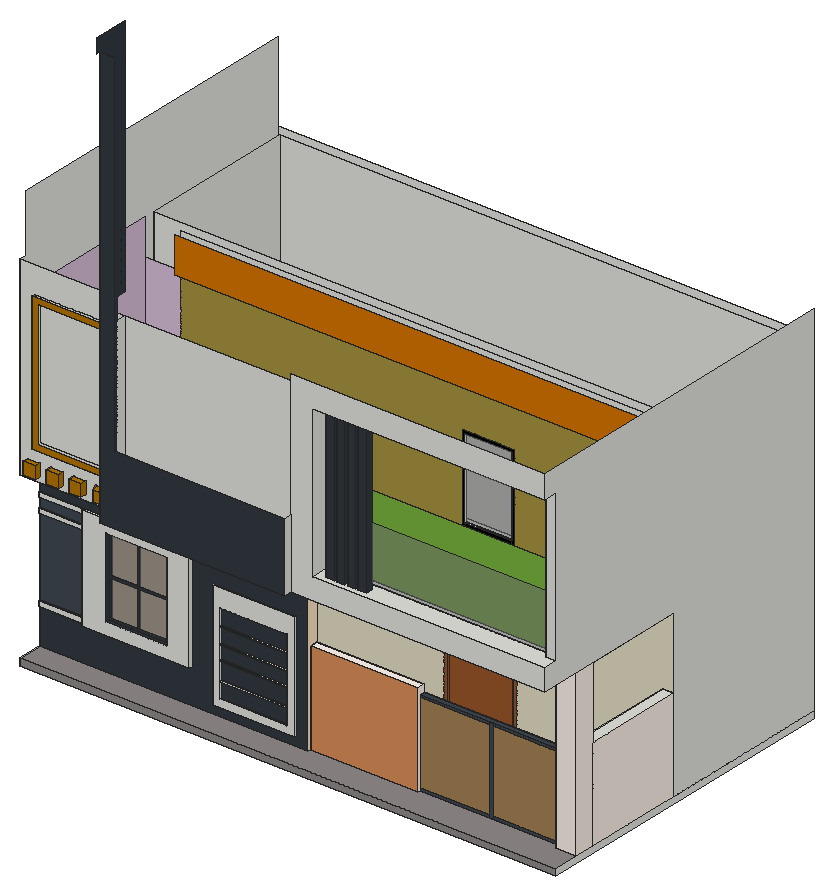
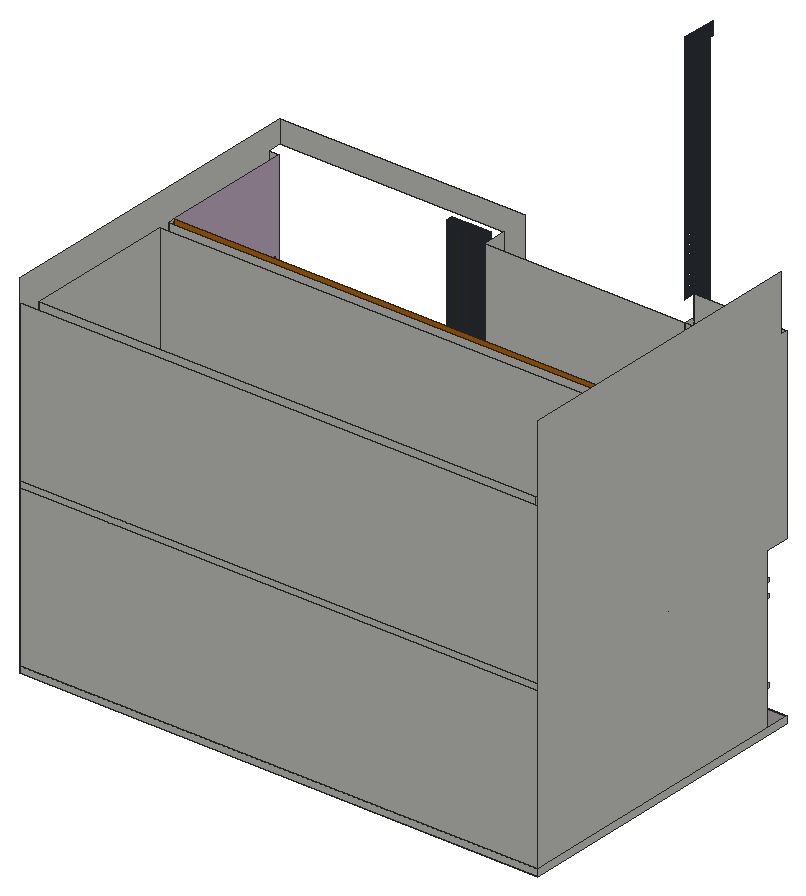
# SketchUp Ruby script. Lengths in inches.
U = 1.inch
M = Sketchup.active_model
def pt(a) = Geom::Point3d.new(a.map { |v| v * U })
def face(e, loops, mat)
  f = e.add_face(loops[0].map { |a| pt(a) })
  loops[1..].each { |l| e.add_face(l.map { |a| pt(a) }).erase! }
  f.material = f.back_material = mat if mat
  f
end
# faces: each face lists its corners as indices into pts; further lists are holes
def faces(e, pts, list, mat = nil) = list.each { |f| face(e, (f[0].is_a?(Array) ? f : [f]).map { |l| l.map { |i| pts[i] } }, mat) }
# xy, xz, yz: faces in a plane at the given z, y or x. An outline is a flat list of corners, or four numbers for a rectangle; further outlines are holes
def ring(l) = l.size == 4 ? [[l[0], l[1]], [l[2], l[1]], [l[2], l[3]], [l[0], l[3]]] : l.each_slice(2).to_a
def flat(e, list, mat, &to3) = list.each { |f| face(e, (f[0].is_a?(Array) ? f : [f]).map { |l| ring(l).map { |u, v| to3.(u, v) } }, mat) }
def xy(e, z, list, mat = nil) = flat(e, list, mat) { |x, y| [x, y, z] }
def xz(e, y, list, mat = nil) = flat(e, list, mat) { |x, z| [x, y, z] }
def yz(e, x, list, mat = nil) = flat(e, list, mat) { |y, z| [x, y, z] }
def lines(e, pts, list) = list.each { |a, b| e.add_line(pt(pts[a]), pt(pts[b])) }
# prism: a flat outline (further loops are holes) pulled along v
def prism(e, loops, v, mat = nil)
  f = face(e, loops, mat); d = Geom::Vector3d.new(v.map { |x| x * U })
  f.pushpull(f.normal.samedirection?(d) ? d.length : -d.length)
end
def box(e, o, s, mat = nil) = prism(e, [[o, [o[0] + s[0], o[1], o[2]], [o[0] + s[0], o[1] + s[1], o[2]], [o[0], o[1] + s[1], o[2]]]], [0, 0, s[2]], mat)
def at(x, y, z, deg = 0) = Geom::Transformation.translation(pt([x, y, z])) * Geom::Transformation.rotation(ORIGIN, Z_AXIS, deg.degrees)
def axes(o, x, y, z) = Geom::Transformation.new([*x, 0, *y, 0, *z, 0, *pt(o).to_a, 1])
def part(name) = M.definitions.add(name)
# library, detail: a bought-in or finely detailed component or shape, given as its bounding box
def library(name, o, s) = part(name).tap { |d| box(d.entities, o, s) }
def detail(e, o, s) = box(e.add_group.entities, o, s)
def put(e, d, t, mat = nil) = e.add_instance(d, t).tap { |i| i.material = mat if mat }
def group(e, t, mat = nil) = e.add_group.tap { |g| g.transformation = t; g.material = mat if mat }.entities
root = M.entities
M.materials.add("[0009_Linen]").color = [250, 240, 230]
M.materials.add("[0011_Seashell]").color = [255, 245, 238]
M.materials.add("[0012_Bisque]").color = [186, 166, 143]
M.materials.add("[0012_Bisque]1").color = [255, 228, 196]
M.materials.add("[0038_Orange]").color = [181, 117, 0]
M.materials.add("[0039_DarkOrange]").color = [214, 117, 0]
M.materials.add("[0051_Cornsilk]").color = [226, 220, 195]
M.materials.add("[0111_SlateGray]").color = [51, 58, 66]
M.materials.add("[0111_SlateGray]2").color = [63, 72, 81]
M.materials.add("[0116_Lavender]").color = [230, 230, 250]
M.materials.add("[0118_Thistle]").color = [216, 191, 216]
M.materials.add("[0137_Black]").color = [0, 0, 0]
M.materials.add("[Beadboard]").color = [218, 143, 90]
M.materials.add("[Granite Brown]").color = [126, 104, 91]
M.materials.add("[Grass Dark Green]").color = [106, 157, 55]
M.materials.add("[Modern Siding]").color = [163, 129, 83]
M.materials.add("[Stone Coursed Rough]").color = [165, 147, 63]
M.materials.add("[Stone Marble]").color = [143, 138, 136]
M.materials.add("[Translucent Glass Gray]").color = [128, 128, 128]
M.materials["[Translucent Glass Gray]"].alpha = 0.5
M.materials.add("[Wood Cherry Original]").color = [152, 86, 42]
xy(root,0,[[0,138,900,678]])
xy(root,12,[[0,180,18,396],[18,180,450,198],[865.875,180,900,214.125],[450,185,630,198],[630,189,865.875,198],
  [882,214.125,900,384],[882,384,882,660,18,660,18,396,0,396,0,678,900,678,900,384],[18,384,882,396],[18,396,882,660]])
xy(root,12,[[18,198,865.875,198,865.875,214.125,882,214.125,882,384,18,384]],"[Granite Brown]")
xy(root,12,[[0,138,900,138,900,180,865.875,180,865.875,189,630,189,630,185,450,185,450,180,0,180]],"[Stone Marble]")
xy(root,19.46,[[521.75,384,630.34,386]],"[Wood Cherry Original]")
xy(root,27.77,[[292.08,177,429.33,180]])
xy(root,39.77,[[304.08,177,417.33,180]])
xy(root,66.37,[[304.08,177,417.33,180]])
xy(root,68.32,[[304.08,177,417.33,180]])
xy(root,70.46,[[74.4,174,254.15,180]])
xy(root,73.28,[[0,177,74.4,180]])
xy(root,81.37,[[0,177,74.4,180]])
xy(root,91.52,[[115.89,174,217.33,180]],"[0111_SlateGray]")
xy(root,96.88,[[304.08,177,417.33,180]])
xy(root,98.83,[[304.08,177,417.33,180]])
xy(root,121.13,[[304.08,177,417.33,180]])
xy(root,123.08,[[304.08,177,417.33,180]])
xy(root,148.13,[[304.08,177,417.33,180]])
xy(root,150.08,[[304.08,177,417.33,180]])
xy(root,156,[[630,189,865.875,198]],"[0111_SlateGray]2")
xy(root,168,[[882,214.125,900,384]])
xy(root,168,[[450,185,630,198]],"[0011_Seashell]")
xy(root,177.77,[[304.08,177,417.33,180]])
xy(root,204.37,[[521.75,384,630.34,386]],"[Wood Cherry Original]")
xy(root,207.77,[[292.08,177,429.33,180]])
xy(root,213.2,[[0,177,74.4,180]])
xy(root,220.36,[[0,177,74.4,180]])
xy(root,224.58,[[115.89,174,217.33,180]],"[0111_SlateGray]")
xy(root,237.75,[[0,177,74.4,180]])
xy(root,244.84,[[74.4,174,254.15,180],[0,177,74.4,180]])
xy(root,288,[[18,384,882,396],[18,396,882,660]])
xy(root,288,[[[162,102,162,138,0,138,0,180,450,180,450,198,18,198,18,384,900,384,900,214.125,865.875,214.125,865.875,180,900,180,900,114,474,114,474,102],[627.41,194.94,630.54,194.97,633.5625,195.81,636.26,197.39,638.46,199.63,640,202.35,640.79,205.39,640.76,208.52,639.93,211.54,638.34,214.24,636.1,216.43,633.38,217.98,630.35,218.76,627.21,218.74,624.19,217.9,621.49,216.3125,619.3,214.08,617.75,211.36,616.97,208.32,616.99,205.19,617.83,202.17,619.42,199.47,621.65,197.27,624.375,195.73],[507.41,194.94,510.54,194.97,513.5625,195.81,516.26,197.39,518.46,199.63,520,202.35,520.79,205.39,520.76,208.52,519.93,211.54,518.34,214.24,516.1,216.43,513.38,217.98,510.35,218.76,507.21,218.74,504.19,217.9,501.49,216.3125,499.3,214.08,497.75,211.36,496.97,208.32,496.99,205.19,497.83,202.17,499.42,199.47,501.65,197.27,504.375,195.73],[747.41,194.94,750.54,194.97,753.5625,195.81,756.26,197.39,758.46,199.63,760,202.35,760.79,205.39,760.76,208.52,759.93,211.54,758.34,214.24,756.1,216.43,753.38,217.98,750.35,218.76,747.21,218.74,744.19,217.9,741.49,216.3125,739.3,214.08,737.75,211.36,736.97,208.32,736.99,205.19,737.83,202.17,739.42,199.47,741.65,197.27,744.375,195.73]],[507.41,194.94,504.375,195.73,501.65,197.27,499.42,199.47,497.83,202.17,496.99,205.19,496.97,208.32,497.75,211.36,499.3,214.08,501.49,216.3125,504.19,217.9,507.21,218.74,510.35,218.76,513.38,217.98,516.1,216.43,518.34,214.24,519.93,211.54,520.76,208.52,520.79,205.39,520,202.35,518.46,199.63,516.26,197.39,513.5625,195.81,510.54,194.97],[627.41,194.94,624.375,195.73,621.65,197.27,619.42,199.47,617.83,202.17,616.99,205.19,616.97,208.32,617.75,211.36,619.3,214.08,621.49,216.3125,624.19,217.9,627.21,218.74,630.35,218.76,633.38,217.98,636.1,216.43,638.34,214.24,639.93,211.54,640.76,208.52,640.79,205.39,640,202.35,638.46,199.63,636.26,197.39,633.5625,195.81,630.54,194.97],[747.41,194.94,744.375,195.73,741.65,197.27,739.42,199.47,737.83,202.17,736.99,205.19,736.97,208.32,737.75,211.36,739.3,214.08,741.49,216.3125,744.19,217.9,747.21,218.74,750.35,218.76,753.38,217.98,756.1,216.43,758.34,214.24,759.93,211.54,760.76,208.52,760.79,205.39,760,202.35,758.46,199.63,756.26,197.39,753.5625,195.81,750.54,194.97]],"[0116_Lavender]")
xy(root,296.37,[[12.68,129,33.18,138],[51.08,129,71.58,138],[89.48,129,109.98,138],[129.52,129,127.875,138,148.375,138,148.375,129]],"[0038_Orange]")
xy(root,300,[[822,366,882,378],[18,396,882,660]])
xy(root,300,[[18,156,882,156,882,366,822,366,822,378,18,378]],"[Grass Dark Green]")
xy(root,305.36,[[554.68,378,633.07,380]])
xy(root,316.87,[[12.68,129,33.18,138],[51.08,129,71.58,138],[89.48,129,109.98,138]],"[0038_Orange]")
xy(root,324,[[[510,114,900,114,900,138,882,138,882,147,510,147],[524.46,124.29,538.65,136.29],[542.46,124.29,556.65,136.29],[560.46,124.29,574.65,136.29],[578.46,124.29,592.65,136.29]],[524.46,124.29,538.65,136.29],[542.46,124.29,556.65,136.29],[560.46,124.29,574.65,136.29],[578.46,124.29,592.65,136.29],
  [510,147,882,156]])
xy(root,338.14,[[25.18,132,152.37,138]],"[0038_Orange]")
xz(root,102,[[162,288,474,288,474,404.14,186,404.14,186,996,162,996]],"[0111_SlateGray]")
xz(root,114,[[474,288,900,288,900,324,510,324,510,576,900,576,900,615.875,474,615.875]])
xz(root,124.29,[[524.46,324,538.65,576],[542.46,324,556.65,576],[560.46,324,574.65,576],[578.46,324,592.65,576]],"[0111_SlateGray]")
xz(root,129,[[12.68,296.37,33.18,316.87],[51.08,296.37,71.58,316.87],[89.48,296.37,109.98,316.87],[129.52,296.37,148.375,315.23]],"[0038_Orange]")
xz(root,132,[[[25.18,338.14,152.37,567.51],[34.01,346.96,143.55,558.6875]]],"[0038_Orange]")
xz(root,136.29,[[524.46,324,538.65,576],[542.46,324,556.65,576],[560.46,324,574.65,576],[578.46,324,592.65,576]],"[0111_SlateGray]")
xz(root,138,[[[0,288,162,612],[25.18,338.14,152.37,567.51],[12.68,296.37,33.18,316.87],[51.08,296.37,71.58,316.87],[89.48,296.37,109.98,316.87],[127.875,296.37,148.375,316.87]],[127.875,296.37,148.375,316.87],[882,324,900,576],[[25.18,338.14,152.37,567.51],[34.01,346.96,143.55,558.6875]]])
xz(root,138,[[0,0,900,12]],"[Stone Marble]")
xz(root,147,[[510,324,882,417]],"[Translucent Glass Gray]")
xz(root,156,[[18,300,162,576],[162,300,510,576],[510,300,882,324]])
xz(root,174,[[[74.4,70.46,254.15,244.84],[115.89,91.52,217.33,224.58]]])
xz(root,177,[[[292.08,27.77,429.33,207.77],[304.08,39.77,417.33,177.77]],[304.08,66.37,417.33,68.32],[0,73.28,74.4,81.37],[304.08,96.88,417.33,98.83],[304.08,121.13,417.33,123.08],
  [304.08,148.13,417.33,150.08],[0,213.2,74.4,220.36],[0,237.75,74.4,244.84]])
xz(root,180,[[[292.08,27.77,429.33,207.77],[304.08,39.77,417.33,177.77]],[[74.4,70.46,254.15,244.84],[115.89,91.52,217.33,224.58]],[0,73.28,74.4,81.37],[0,213.2,74.4,220.36],[0,237.75,74.4,244.84]])
xz(root,180,[[865.875,12,900,288]],"[0009_Linen]")
xz(root,180,[[[0,12,450,12,450,288,0,288,0,244.84,254.15,244.84,254.15,70.46,74.4,70.46,74.4,73.28,0,73.28],[292.08,27.77,429.33,207.77]],[304.08,39.77,417.33,66.37],[304.08,68.32,417.33,96.88],[[115.89,91.52,217.33,224.58],[119.83,95.46,213.38,220.64]],[164.78,95.46,168.08,155.49],
  [304.08,98.83,417.33,121.13],[304.08,123.08,417.33,148.13],[304.08,150.08,417.33,177.77],[119.83,155.49,164.78,159.39],[164.78,155.49,168.08,159.39],
  [168.08,155.49,213.38,159.39],[164.78,159.39,168.08,220.64]],"[0111_SlateGray]")
xz(root,180,[[0,81.37,74.4,213.2],[0,220.36,74.4,237.75]],"[0111_SlateGray]2")
xz(root,180,[[119.83,95.46,164.78,155.49],[168.08,95.46,213.38,155.49],[119.83,159.39,164.78,220.64],[168.08,159.39,213.38,220.64]],"[Translucent Glass Gray]")
xz(root,185,[[450,12,630,168]],"[Beadboard]")
xz(root,189,[[630,12,746.93,16.45],[746.93,12,752.1,156],[752.1,12,865.875,16.45],[630,151.97,746.93,156],[752.1,151.97,865.875,156]],"[0111_SlateGray]2")
xz(root,189,[[630,16.45,746.93,151.97],[752.1,16.45,865.875,151.97]],"[Modern Siding]")
xz(root,198,[[18,12,450,288]],"[0012_Bisque]")
xz(root,198,[[450,12,630,168]],"[Beadboard]")
xz(root,198,[[630,12,865.875,156]],"[Modern Siding]")
xz(root,214.125,[[882,12,900,168]])
xz(root,214.125,[[865.875,12,865.875,288,900,288,900,168,882,168,882,12]],"[0011_Seashell]")
xz(root,366,[[822,300,882,300,882,576,78,576,78,516,822,516]],"[0039_DarkOrange]")
xz(root,378,[[822,300,822,516,78,516,78,576,882,576,882,300]])
xz(root,378,[[18,300,78,516]],"[0118_Thistle]")
xz(root,378,[[549.3125,300,554.68,300,554.68,438.84,633.07,438.84,633.07,300,638.4375,300,638.4375,444.21,549.3125,444.21],[554.68,300,633.07,305.36]],"[0137_Black]")
xz(root,378,[[78,300,549.3125,300,549.3125,444.21,638.4375,444.21,638.4375,300,822,300,822,516,78,516]],"[Stone Coursed Rough]")
xz(root,380,[[554.68,305.36,633.07,438.84]],"[Translucent Glass Gray]")
xz(root,384,[[882,12,900,168]])
xz(root,384,[[18,12,514.29,12,514.29,211.83,637.79,211.83,637.79,12,882,12,882,168,900,168,900,288,18,288]],"[0051_Cornsilk]")
xz(root,384,[[[514.29,12,637.79,211.83],[521.75,19.46,630.34,204.37]]],"[Wood Cherry Original]")
xz(root,386,[[521.75,19.46,630.34,204.37]],"[Wood Cherry Original]")
xz(root,396,[[18,12,882,288],[18,300,882,576]])
xz(root,660,[[18,12,882,288],[18,300,882,576]])
xz(root,678,[[0,0,900,12],[0,12,900,288],[0,288,900,300],[0,300,900,576]])
yz(root,0,[[138,0,678,12],[180,12,180,288,138,288,138,612,149.68,612,149.68,709.65,678,709.65,678,12],[177,73.28,180,81.37],[177,213.2,180,220.36],[177,237.75,180,244.84]])
yz(root,12.68,[[129,296.37,138,316.87]],"[0038_Orange]")
yz(root,18,[[384,12,396,288],[396,12,660,288],[396,300,660,576]])
yz(root,18,[[198,12,384,288]],"[0012_Bisque]")
yz(root,18,[[156,300,378,576]],"[0118_Thistle]")
yz(root,25.18,[[132,338.14,138,567.51]],"[0038_Orange]")
yz(root,33.18,[[129,296.37,138,316.87]],"[0038_Orange]")
yz(root,51.08,[[129,296.37,138,316.87]],"[0038_Orange]")
yz(root,71.58,[[129,296.37,138,316.87]],"[0038_Orange]")
yz(root,74.4,[[174,70.46,174,244.84,177,244.84,177,237.75,180,237.75,180,220.36,177,220.36,177,213.2,180,213.2,180,81.37,177,81.37,177,73.28,180,73.28,180,70.46],[177,73.28,180,81.37],[177,213.2,180,220.36],[177,237.75,180,244.84]])
yz(root,89.48,[[129,296.37,138,316.87]],"[0038_Orange]")
yz(root,109.98,[[129,296.37,138,316.87]],"[0038_Orange]")
yz(root,115.89,[[174,91.52,180,224.58]],"[0111_SlateGray]")
yz(root,148.375,[[129,296.37,138,296.37,138,316.87,129,315.23]],"[0038_Orange]")
yz(root,152.37,[[132,338.14,138,567.51]],"[0038_Orange]")
yz(root,162,[[138,300,156,576]])
yz(root,162,[[[102,288,102,996,96,996,96,1020,156,1020,156,612,138,612,138,288],[146.77,660.69,147,660.7,147.55,660.73,148.3,660.98,148.95,661.41,149.48,661.99,149.83,662.6875,149.99,663.45,149.95,664.24,149.71,664.98,149.28,665.64,148.69,666.16,148,666.51,147.23,666.67,147,666.66,146.45,666.63,145.7,666.39,145.05,665.96,144.52,665.375,144.17,664.68,144.01,663.91,144.05,663.13,144.29,662.39,144.72,661.73,145.31,661.21,146,660.85],[146.625,675.5,147,675.5,147.41,675.51,148.16,675.71,148.84,676.11,149.39,676.67,149.78,677.35,149.98,678.1,149.97,678.89,149.76,679.64,149.37,680.32,148.8125,680.87,148.13,681.26,147.375,681.45,146.59,681.45,145.84,681.24,145.16,680.85,144.61,680.29,144.22,679.61,144.02,678.85,144.03,678.07,144.24,677.3125,144.63,676.64,145.1875,676.09,145.87,675.7],[146.6,625.86,147.38,625.86,148.14,626.06,148.82,626.45,149.37,627,149.77,627.68,149.97,628.43,149.98,629.21,149.78,629.97,149.39,630.65,148.84,631.21,148.16,631.6,147.4,631.81,147,631.81,146.62,631.8125,145.86,631.61,145.18,631.22,144.63,630.67,144.23,629.99,144.03,629.24,144.02,628.46,144.22,627.7,144.61,627.02,145.16,626.46,145.84,626.07],[147,690.27,147.78,690.375,148.5,690.68,149.12,691.15,149.6,691.77,149.9,692.5,150,693.27,149.9,694.05,149.6,694.77,149.12,695.4,148.5,695.87,147.78,696.17,147,696.27,146.22,696.17,145.5,695.87,144.88,695.4,144.4,694.77,144.1,694.05,144,693.27,144.1,692.5,144.4,691.77,144.88,691.15,145.5,690.68,146.22,690.375],[146.96,643.48,147,643.48,147.74,643.57,148.47,643.86,149.09,644.33,149.58,644.95,149.89,645.66,150,646.44,149.91,647.22,149.62,647.95,149.15,648.57,148.53,649.06,147.82,649.37,147.04,649.48,147,649.47,146.26,649.39,145.53,649.1,144.91,648.63,144.42,648.01,144.11,647.3,144,646.52,144.09,645.74,144.38,645.01,144.85,644.39,145.47,643.9,146.18,643.59],[146.82,705.01,147,705.02,147.6,705.0625,148.34,705.32,148.99,705.76,149.5,706.35,149.85,707.05,149.99,707.82,149.9375,708.6,149.68,709.34,149.24,709.99,148.65,710.5,147.95,710.85,147.18,710.99,146.4,710.9375,145.66,710.68,145.01,710.24,144.5,709.65,144.15,708.95,144.01,708.18,144.0625,707.4,144.32,706.66,144.76,706.01,145.35,705.5,146.05,705.15]]],"[0111_SlateGray]")
yz(root,217.33,[[174,91.52,180,224.58]],"[0111_SlateGray]")
yz(root,254.15,[[174,70.46,180,244.84]])
yz(root,292.08,[[177,27.77,180,207.77]])
yz(root,304.08,[[177,39.77,180,66.37],[177,66.37,180,68.32],[177,68.32,180,96.88],[177,96.88,180,98.83],[177,98.83,180,121.13],
  [177,121.13,180,123.08],[177,123.08,180,148.13],[177,148.13,180,150.08],[177,150.08,180,177.77]])
yz(root,417.33,[[177,39.77,180,66.37],[177,66.37,180,68.32],[177,68.32,180,96.88],[177,96.88,180,98.83],[177,98.83,180,121.13],
  [177,121.13,180,123.08],[177,123.08,180,148.13],[177,148.13,180,150.08],[177,150.08,180,177.77]])
yz(root,429.33,[[177,27.77,180,207.77]])
yz(root,450,[[185,12,198,168]])
yz(root,450,[[180,12,185,12,185,168,198,168,198,288,180,288]],"[0012_Bisque]1")
yz(root,474,[[102,288,114,404.14]])
yz(root,510,[[114,324,147,324,147,417,146.22,417.1,145.5,417.4,144.88,417.88,144.4,418.5,144.1,419.22,144,420,144.1,420.78,144.4,421.5,144.88,422.12,145.5,422.6,146.22,422.9,147,423,147.78,422.9,148.5,422.6,149.12,422.12,149.6,421.5,149.9,420.78,150,420,149.9,419.22,149.6,418.5,149.12,417.88,148.5,417.4,147.78,417.1,147,417,147,324,156,324,156,576,114,576]])
yz(root,521.75,[[384,19.46,386,204.37]],"[Wood Cherry Original]")
yz(root,524.46,[[124.29,324,136.29,576]],"[0111_SlateGray]")
yz(root,538.65,[[124.29,324,136.29,576]],"[0111_SlateGray]")
yz(root,542.46,[[124.29,324,136.29,576]],"[0111_SlateGray]")
yz(root,554.68,[[378,305.36,380,438.84]])
yz(root,556.65,[[124.29,324,136.29,576]],"[0111_SlateGray]")
yz(root,560.46,[[124.29,324,136.29,576]],"[0111_SlateGray]")
yz(root,574.65,[[124.29,324,136.29,576]],"[0111_SlateGray]")
yz(root,578.46,[[124.29,324,136.29,576]],"[0111_SlateGray]")
yz(root,592.65,[[124.29,324,136.29,576]],"[0111_SlateGray]")
yz(root,630,[[189,12,198,156]])
yz(root,630,[[185,12,189,12,189,156,198,156,198,168,185,168]],"[0011_Seashell]")
yz(root,630.34,[[384,19.46,386,204.37]],"[Wood Cherry Original]")
yz(root,633.07,[[378,305.36,380,438.84]])
yz(root,822,[[366,300,378,516]],"[0039_DarkOrange]")
yz(root,865.875,[[189,12,198,156]])
yz(root,865.875,[[180,12,180,288,214.125,288,214.125,12,198,12,198,156,189,156,189,12]],"[0009_Linen]")
yz(root,882,[[214.125,12,384,168],[396,12,660,288],[366,300,378,576],[396,300,660,576]])
yz(root,882,[[156,300,156,324,147,324,147,417,147.78,417.1,148.5,417.4,149.12,417.88,149.6,418.5,149.9,419.22,150,420,149.9,420.78,149.6,421.5,149.12,422.12,148.5,422.6,147.78,422.9,147,423,146.22,422.9,145.5,422.6,144.88,422.12,144.4,421.5,144.1,420.78,144,420,144.1,419.22,144.4,418.5,144.88,417.88,145.5,417.4,146.22,417.1,147,417,147,324,138,324,138,576,366,576,366,300]],"[0118_Thistle]")
yz(root,900,[[138,0,678,12],[384,12,678,12,678,615.875,114,615.875,114,576,138,576,138,324,114,324,114,288,384,288]])
yz(root,900,[[180,12,214.125,288],[214.125,12,384,168]],"[0009_Linen]")
p = [[129.52,129,315.23],[127.875,138,316.87],[127.875,138,296.37],[129.52,129,296.37],[148.375,129,315.23],[148.375,138,316.87],
  [18,396,288],[0,396,288],[18,180,288],[18,198,288],[18,156,300],[18,138,300]]
faces(root,p,[[0,1,2,3],[0,4,5,1]],"[0038_Orange]")
lines(root,p,[[6,7],[8,9],[10,11]])
